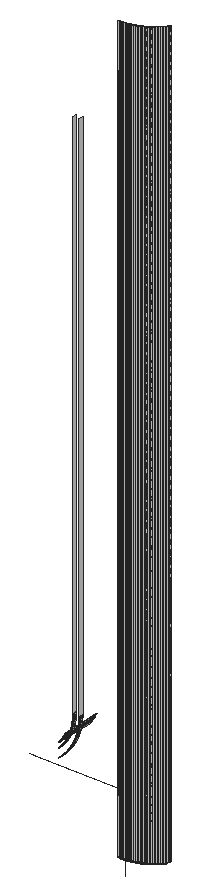
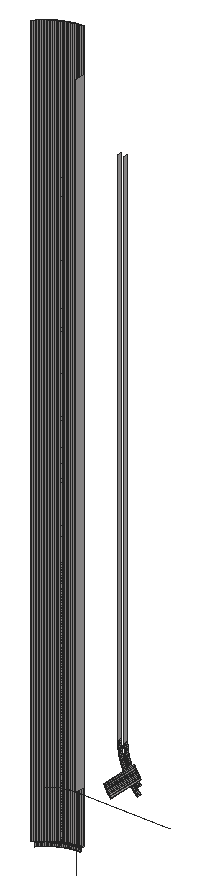
# SketchUp Ruby script. Lengths in inches.
U = 1.inch
M = Sketchup.active_model
def pt(a) = Geom::Point3d.new(a.map { |v| v * U })
def face(e, loops, mat)
  f = e.add_face(loops[0].map { |a| pt(a) })
  loops[1..].each { |l| e.add_face(l.map { |a| pt(a) }).erase! }
  f.material = f.back_material = mat if mat
  f
end
# faces: each face lists its corners as indices into pts; further lists are holes
def faces(e, pts, list, mat = nil) = list.each { |f| face(e, (f[0].is_a?(Array) ? f : [f]).map { |l| l.map { |i| pts[i] } }, mat) }
# xy, xz, yz: faces in a plane at the given z, y or x. An outline is a flat list of corners, or four numbers for a rectangle; further outlines are holes
def ring(l) = l.size == 4 ? [[l[0], l[1]], [l[2], l[1]], [l[2], l[3]], [l[0], l[3]]] : l.each_slice(2).to_a
def flat(e, list, mat, &to3) = list.each { |f| face(e, (f[0].is_a?(Array) ? f : [f]).map { |l| ring(l).map { |u, v| to3.(u, v) } }, mat) }
def xy(e, z, list, mat = nil) = flat(e, list, mat) { |x, y| [x, y, z] }
def xz(e, y, list, mat = nil) = flat(e, list, mat) { |x, z| [x, y, z] }
def yz(e, x, list, mat = nil) = flat(e, list, mat) { |y, z| [x, y, z] }
def lines(e, pts, list) = list.each { |a, b| e.add_line(pt(pts[a]), pt(pts[b])) }
# prism: a flat outline (further loops are holes) pulled along v
def prism(e, loops, v, mat = nil)
  f = face(e, loops, mat); d = Geom::Vector3d.new(v.map { |x| x * U })
  f.pushpull(f.normal.samedirection?(d) ? d.length : -d.length)
end
def box(e, o, s, mat = nil) = prism(e, [[o, [o[0] + s[0], o[1], o[2]], [o[0] + s[0], o[1] + s[1], o[2]], [o[0], o[1] + s[1], o[2]]]], [0, 0, s[2]], mat)
def at(x, y, z, deg = 0) = Geom::Transformation.translation(pt([x, y, z])) * Geom::Transformation.rotation(ORIGIN, Z_AXIS, deg.degrees)
def axes(o, x, y, z) = Geom::Transformation.new([*x, 0, *y, 0, *z, 0, *pt(o).to_a, 1])
def part(name) = M.definitions.add(name)
# library, detail: a bought-in or finely detailed component or shape, given as its bounding box
def library(name, o, s) = part(name).tap { |d| box(d.entities, o, s) }
def detail(e, o, s) = box(e.add_group.entities, o, s)
def put(e, d, t, mat = nil) = e.add_instance(d, t).tap { |i| i.material = mat if mat }
def group(e, t, mat = nil) = e.add_group.tap { |g| g.transformation = t; g.material = mat if mat }.entities
root = M.entities
M.materials.add("[Quartz Light Brown]").color = [215, 212, 212]
xz(root,143,[[480,133,480.2,368]],"[Quartz Light Brown]")
xz(root,143.01,[[480.39,133,480.59,368]],"[Quartz Light Brown]")
xz(root,144,[[480,132,480.18,133],[480.18,132,480.37,133]],"[Quartz Light Brown]")
yz(root,465.99,[[143,167.37,144.25,167.58]],"[Quartz Light Brown]")
yz(root,466,[[143,167.79,144.25,168],[143,168,144.25,336]],"[Quartz Light Brown]")
yz(root,467.99,[[143,167.29,144.25,167.53]],"[Quartz Light Brown]")
yz(root,468,[[143,167.76,144.25,168],[143,168,144.25,336]],"[Quartz Light Brown]")
yz(root,480,[[143,150,146,354]],"[Quartz Light Brown]")
p = [[480.37,144,133],[480.37,144,132],[480.55,144.01,132],[480.55,144.01,133],[480.73,144.02,132],[480.73,144.02,133],
  [480.92,144.03,132],[480.92,144.03,133],[481.1,144.04,132],[481.1,144.04,133],[481.28,144.06,132],[481.28,144.06,133],
  [481.46,144.08,132],[481.46,144.08,133],[481.65,144.1,132],[481.65,144.1,133],[481.83,144.12,132],[481.83,144.12,133],
  [482.01,144.14,132],[482.01,144.14,133],[482.19,144.17,132],[482.19,144.17,133],[482.37,144.2,132],[482.37,144.2,133],
  [482.55,144.23,132],[482.55,144.23,133],[482.73,144.27,132],[482.73,144.27,133],[482.91,144.31,132],[482.91,144.31,133],
  [483.09,144.35,132],[483.09,144.35,133],[483.27,144.39,132],[483.27,144.39,133],[483.45,144.43,132],[483.45,144.43,133],
  [483.625,144.48,132],[483.625,144.48,133],[483.8,144.53,132],[483.8,144.53,133],[483.98,144.58,132],[483.98,144.58,133],
  [484.15,144.63,132],[484.15,144.63,133],[484.33,144.69,132],[484.33,144.69,133],[484.5,144.74,132],[484.5,144.74,133],
  [484.67,144.8,132],[484.67,144.8,133],[484.85,144.87,132],[484.85,144.87,133],[485.02,144.93,132],[485.02,144.93,133],
  [485.1875,145,132],[485.1875,145,133],[485.36,145.07,132],[485.36,145.07,133],[485.53,145.14,132],[485.53,145.14,133],
  [485.69,145.21,132],[485.69,145.21,133],[485.86,145.29,132],[485.86,145.29,133],[486.03,145.36,132],[486.03,145.36,133],
  [486.19,145.44,132],[486.19,145.44,133],[486.36,145.53,132],[486.36,145.53,133],[486.52,145.61,132],[486.52,145.61,133],
  [486.68,145.7,132],[486.68,145.7,133],[486.84,145.79,132],[486.84,145.79,133],[487,145.875,132],[487,145.875,133],
  [487.16,145.97,132],[487.16,145.97,133],[487.31,146.0625,132],[487.31,146.0625,133],[487.47,146.16,132],[487.47,146.16,133],
  [487.625,146.26,132],[487.625,146.26,133],[487.78,146.36,132],[487.78,146.36,133],[487.93,146.46,132],[487.93,146.46,133],
  [488.08,146.57,132],[488.08,146.57,133],[488.23,146.67,132],[488.23,146.67,133],[488.375,146.78,132],[488.375,146.78,133],
  [488.52,146.89,132],[488.52,146.89,133],[488.67,147.01,132],[488.67,147.01,133],[488.81,147.12,132],[488.81,147.12,133],
  [488.95,147.24,132],[488.95,147.24,133],[489.09,147.35,132],[489.09,147.35,133],[489.23,147.47,132],[489.23,147.47,133],
  [489.37,147.6,132],[489.37,147.6,133],[489.5,147.72,132],[489.5,147.72,133],[489.64,147.84,132],[489.64,147.84,133],
  [489.77,147.97,132],[489.77,147.97,133],[489.9,148.1,132],[489.9,148.1,133],[490.03,148.23,132],[490.03,148.23,133],
  [490.16,148.36,132],[490.16,148.36,133],[490.28,148.5,132],[490.28,148.5,133],[490.4,148.63,132],[490.4,148.63,133],
  [490.53,148.77,132],[490.53,148.77,133],[490.65,148.91,132],[490.65,148.91,133],[490.76,149.05,132],[490.76,149.05,133],
  [480.2,143,368],[480.2,143,133],[480.39,143.01,133],[480.39,143.01,368],[480.59,143.01,368],[480.59,143.01,133],
  [480.79,143.02,133],[480.79,143.02,368],[480.98,143.03,133],[480.98,143.03,368],[481.18,143.05,133],[481.18,143.05,368],
  [481.37,143.0625,133],[481.37,143.0625,368],[481.57,143.08,133],[481.57,143.08,368],[481.76,143.1,133],[481.76,143.1,368],
  [481.96,143.13,133],[481.96,143.13,368],[482.15,143.16,133],[482.15,143.16,368],[482.35,143.18,133],[482.35,143.18,368],
  [482.54,143.22,133],[482.54,143.22,368],[482.73,143.25,133],[482.73,143.25,368],[482.93,143.29,133],[482.93,143.29,368],
  [483.12,143.33,133],[483.12,143.33,368],[483.31,143.37,133],[483.31,143.37,368],[483.5,143.41,133],[483.5,143.41,368],
  [483.69,143.46,133],[483.69,143.46,368],[483.88,143.51,133],[483.88,143.51,368],[484.07,143.5625,133],[484.07,143.5625,368],
  [484.26,143.62,133],[484.26,143.62,368],[484.45,143.67,133],[484.45,143.67,368],[484.64,143.73,133],[484.64,143.73,368],
  [484.82,143.8,133],[484.82,143.8,368],[485.01,143.86,133],[485.01,143.86,368],[485.19,143.93,133],[485.19,143.93,368],
  [485.375,144,133],[485.375,144,368],[485.56,144.07,133],[485.56,144.07,368],[485.74,144.14,133],[485.74,144.14,368],
  [485.92,144.22,133],[485.92,144.22,368],[486.1,144.3,133],[486.1,144.3,368],[486.28,144.38,133],[486.28,144.38,368],
  [486.46,144.46,133],[486.46,144.46,368],[486.63,144.55,133],[486.63,144.55,368],[486.81,144.63,133],[486.81,144.63,368],
  [486.98,144.73,133],[486.98,144.73,368],[487.16,144.82,133],[487.16,144.82,368],[487.33,144.91,133],[487.33,144.91,368],
  [487.5,145.01,133],[487.5,145.01,368],[487.67,145.11,133],[487.67,145.11,368],[487.84,145.21,133],[487.84,145.21,368],
  [488,145.3125,133],[488,145.3125,368],[488.17,145.42,133],[488.17,145.42,368],[488.33,145.53,133],[488.33,145.53,368],
  [488.5,145.64,133],[488.5,145.64,368],[488.66,145.75,133],[488.66,145.75,368],[488.82,145.86,133],[488.82,145.86,368],
  [488.97,145.98,133],[488.97,145.98,368],[489.13,146.1,133],[489.13,146.1,368],[489.29,146.22,133],[489.29,146.22,368],
  [489.44,146.34,133],[489.44,146.34,368],[489.59,146.47,133],[489.59,146.47,368],[489.74,146.59,133],[489.74,146.59,368],
  [489.89,146.72,133],[489.89,146.72,368],[490.04,146.85,133],[490.04,146.85,368],[490.18,146.99,133],[490.18,146.99,368],
  [490.33,147.12,133],[490.33,147.12,368],[490.47,147.26,133],[490.47,147.26,368],[490.61,147.39,133],[490.61,147.39,368],
  [490.74,147.53,133],[490.74,147.53,368],[490.88,147.67,133],[490.88,147.67,368],[491.01,147.82,133],[491.01,147.82,368],
  [491.15,147.96,133],[491.15,147.96,368],[491.28,148.11,133],[491.28,148.11,368],[491.41,148.26,133],[491.41,148.26,368],
  [491.53,148.41,133],[491.53,148.41,368],[491.66,148.56,133],[491.66,148.56,368],[491.78,148.71,133],[491.78,148.71,368],
  [491.9,148.87,133],[491.9,148.87,368],[492.02,149.03,133],[492.02,149.03,368],[461.69,144.25,154.3125],[461.69,143,154.3125],
  [461.87,143,154.47],[461.87,144.25,154.47],[462.04,143,154.625],[462.04,144.25,154.625],[462.22,143,154.78],[462.22,144.25,154.78],
  [462.39,143,154.94],[462.39,144.25,154.94],[462.56,143,155.11],[462.56,144.25,155.11],[462.73,143,155.27],[462.73,144.25,155.27],
  [462.89,143,155.44],[462.89,144.25,155.44],[463.06,143,155.61],[463.06,144.25,155.61],[463.22,143,155.78],[463.22,144.25,155.78],
  [463.375,143,155.96],[463.375,144.25,155.96],[463.53,143,156.13],[463.53,144.25,156.13],[463.6875,143,156.31],[463.6875,144.25,156.31],
  [463.84,143,156.49],[463.84,144.25,156.49],[463.99,143,156.67],[463.99,144.25,156.67],[464.14,143,156.86],[464.14,144.25,156.86],
  [464.28,143,157.04],[464.28,144.25,157.04],[461.75,143,157.14],[461.61,143,156.99],[461.61,144.25,156.99],[461.75,144.25,157.14],
  [464.42,143,157.23],[464.42,144.25,157.23],[461.89,143,157.29],[461.89,144.25,157.29],[464.5625,143,157.42],[464.5625,144.25,157.42],
  [462.03,143,157.45],[462.03,144.25,157.45],[464.7,143,157.61],[464.7,144.25,157.61],[462.17,143,157.61],[462.17,144.25,157.61],
  [462.3,143,157.77],[462.3,144.25,157.77],[464.83,143,157.8],[464.83,144.25,157.8],[462.43,143,157.93],[462.43,144.25,157.93],
  [464.97,143,158],[464.97,144.25,158],[462.57,143,158.09],[462.57,144.25,158.09],[465.1,143,158.2],[465.1,144.25,158.2],
  [462.69,143,158.26],[462.69,144.25,158.26],[465.22,143,158.39],[465.22,144.25,158.39],[462.82,143,158.43],[462.82,144.25,158.43],
  [462.94,143,158.6],[462.94,144.25,158.6],[465.35,143,158.6],[465.35,144.25,158.6],[461.66,143,158.56],[461.78,143,158.71],
  [461.78,155,158.71],[461.66,155,158.56],[463.07,143,158.77],[463.07,144.25,158.77],[465.47,143,158.8],[465.47,144.25,158.8],
  [461.9,143,158.87],[461.9,155,158.87],[463.1875,143,158.9375],[463.1875,144.25,158.9375],[465.59,143,159],[465.59,144.25,159],
  [462.02,143,159.03],[462.02,155,159.03],[463.3,143,159.11],[463.3,144.25,159.11],[462.14,143,159.18],[462.14,155,159.18],
  [465.7,143,159.2],[465.7,144.25,159.2],[463.42,143,159.29],[463.42,144.25,159.29],[462.25,143,159.34],[462.25,155,159.34],
  [465.82,143,159.41],[465.82,144.25,159.41],[462.36,143,159.5],[462.36,155,159.5],[463.53,143,159.46],[463.53,144.25,159.46],
  [465.93,143,159.62],[465.93,144.25,159.62],[462.47,143,159.67],[462.47,155,159.67],[463.64,143,159.64],[463.64,144.25,159.64],
  [463.75,143,159.82],[463.75,144.25,159.82],[466.04,143,159.83],[466.04,144.25,159.83],[462.58,143,159.83],[462.58,155,159.83],
  [462.6875,143,160],[462.6875,155,160],[463.86,143,160],[463.86,144.25,160],[466.14,143,160.04],[466.14,144.25,160.04],
  [462.79,143,160.16],[462.79,155,160.16],[463.96,143,160.18],[463.96,144.25,160.18],[466.25,143,160.25],[466.25,144.25,160.25],
  [462.89,143,160.33],[462.89,155,160.33],[464.0625,143,160.37],[464.0625,144.25,160.37],[462.99,143,160.5],[462.99,155,160.5],
  [466.35,143,160.46],[466.35,144.25,160.46],[464.16,143,160.55],[464.16,144.25,160.55],[463.09,143,160.67],[463.09,155,160.67],
  [466.44,143,160.68],[466.44,144.25,160.68],[464.26,143,160.74],[464.26,144.25,160.74],[463.18,143,160.84],[463.18,155,160.84],
  [464.35,143,160.92],[464.35,144.25,160.92],[466.54,143,160.89],[466.54,144.25,160.89],[463.27,143,161.02],[463.27,155,161.02],
  [464.44,143,161.11],[464.44,144.25,161.11],[466.63,143,161.11],[466.63,144.25,161.11],[463.37,143,161.19],[463.37,155,161.19],
  [464.53,143,161.3],[464.53,144.25,161.3],[466.72,143,161.33],[466.72,144.25,161.33],[463.45,143,161.37],[463.45,155,161.37],
  [464.62,143,161.49],[464.62,144.25,161.49],[466.8,143,161.55],[466.8,144.25,161.55],[463.54,143,161.54],[463.54,155,161.54],
  [463.62,143,161.72],[463.62,155,161.72],[464.7,143,161.68],[464.7,144.25,161.68],[466.89,143,161.77],[466.89,144.25,161.77],
  [463.7,143,161.9],[463.7,155,161.9],[464.78,143,161.88],[464.78,144.25,161.88],[466.97,143,161.99],[466.97,144.25,161.99],
  [463.78,143,162.08],[463.78,155,162.08],[464.86,143,162.07],[464.86,144.25,162.07],[467.04,143,162.21],[467.04,144.25,162.21],
  [464.9375,143,162.27],[464.9375,144.25,162.27],[467.12,143,162.4375],[467.12,144.25,162.4375],[465.01,143,162.46],[465.01,144.25,162.46],
  [467.19,143,162.66],[467.19,144.25,162.66],[465.08,143,162.66],[465.08,144.25,162.66],[465.15,143,162.86],[465.15,144.25,162.86],
  [467.26,143,162.89],[467.26,144.25,162.89],[465.22,143,163.06],[465.22,144.25,163.06],[467.32,143,163.11],[467.32,144.25,163.11],
  [465.28,143,163.26],[465.28,144.25,163.26],[467.39,143,163.34],[467.39,144.25,163.34],[465.34,143,163.46],[465.34,144.25,163.46],
  [467.45,143,163.57],[467.45,144.25,163.57],[465.4,143,163.66],[465.4,144.25,163.66],[467.5,143,163.8],[467.5,144.25,163.8],
  [465.45,143,163.86],[465.45,144.25,163.86],[467.56,143,164.03],[467.56,144.25,164.03],[465.51,143,164.0625],[465.51,144.25,164.0625],
  [467.61,143,164.26],[467.61,144.25,164.26],[465.56,143,164.26],[465.56,144.25,164.26],[465.61,143,164.47],[465.61,144.25,164.47],
  [467.65,143,164.49],[467.65,144.25,164.49],[465.65,143,164.67],[465.65,144.25,164.67],[467.7,143,164.72],[467.7,144.25,164.72],
  [465.69,143,164.88],[465.69,144.25,164.88],[467.74,143,164.95],[467.74,144.25,164.95],[465.73,143,165.08],[465.73,144.25,165.08],
  [467.78,143,165.18],[467.78,144.25,165.18],[465.77,143,165.29],[465.77,144.25,165.29],[467.8125,143,165.42],[467.8125,144.25,165.42],
  [465.8,143,165.5],[465.8,144.25,165.5],[467.85,143,165.65],[467.85,144.25,165.65],[465.83,143,165.7],[465.83,144.25,165.7],
  [465.86,143,165.91],[465.86,144.25,165.91],[467.875,143,165.88],[467.875,144.25,165.88],[465.89,143,166.12],[465.89,144.25,166.12],
  [467.9,143,166.12],[467.9,144.25,166.12],[465.91,143,166.33],[465.91,144.25,166.33],[467.92,143,166.35],[467.92,144.25,166.35],
  [465.93,143,166.54],[465.93,144.25,166.54],[467.94,143,166.59],[467.94,144.25,166.59],[465.95,143,166.74],[465.95,144.25,166.74],
  [467.96,143,166.82],[467.96,144.25,166.82],[465.97,143,166.95],[465.97,144.25,166.95],[467.98,143,167.06],[467.98,144.25,167.06],
  [465.98,143,167.16],[465.98,144.25,167.16],[467.99,143,167.29],[467.99,144.25,167.29],[465.99,143,167.37],[465.99,144.25,167.37],
  [467.99,144.25,167.53],[467.99,143,167.53],[468,143,167.76],[468,144.25,167.76],[466,143,167.79],[465.99,143,167.58],
  [465.99,144.25,167.58],[466,144.25,167.79],[480,146,150],[480,146,126],[450,146,150],[480.16,146,150],
  [480.3125,146,150],[480.47,146.01,150],[480.63,146.02,150],[480.78,146.03,150],[480.94,146.04,150],[481.1,146.05,150],
  [481.25,146.07,150],[481.41,146.08,150],[481.57,146.1,150],[481.72,146.125,150],[481.88,146.15,150],[482.03,146.17,150],
  [482.1875,146.2,150],[482.34,146.23,150],[482.49,146.26,150],[482.65,146.3,150],[482.8,146.33,150],[482.95,146.37,150],
  [483.11,146.41,150],[483.26,146.45,150],[483.41,146.49,150],[483.56,146.54,150],[483.71,146.59,150],[483.86,146.64,150],
  [484.01,146.6875,150],[484.15,146.74,150],[484.3,146.8,150],[484.45,146.85,150],[484.59,146.91,150],[484.74,146.97,150],
  [484.88,147.04,150],[485.02,147.1,150],[485.17,147.17,150],[485.31,147.24,150],[485.45,147.31,150],[485.59,147.38,150],
  [485.73,147.45,150],[485.86,147.53,150],[486,147.61,150],[486.14,147.6875,150],[486.27,147.77,150],[486.4,147.85,150],
  [486.54,147.9375,150],[486.67,148.02,150],[486.8,148.11,150],[486.93,148.2,150],[487.05,148.29,150],[487.18,148.38,150],
  [487.31,148.48,150],[487.43,148.58,150],[487.55,148.67,150],[487.67,148.77,150],[487.79,148.875,150],[487.91,148.98,150]]
faces(root,p,[[0,1,2,3],[3,2,4,5],[5,4,6,7],[7,6,8,9],[9,8,10,11],[11,10,12,13],[13,12,14,15],[15,14,16,17],
  [17,16,18,19],[19,18,20,21],[21,20,22,23],[23,22,24,25],[25,24,26,27],[27,26,28,29],[29,28,30,31],[31,30,32,33],
  [33,32,34,35],[35,34,36,37],[37,36,38,39],[39,38,40,41],[41,40,42,43],[43,42,44,45],[45,44,46,47],[47,46,48,49],
  [49,48,50,51],[51,50,52,53],[53,52,54,55],[55,54,56,57],[57,56,58,59],[59,58,60,61],[61,60,62,63],[63,62,64,65],
  [65,64,66,67],[67,66,68,69],[69,68,70,71],[71,70,72,73],[73,72,74,75],[75,74,76,77],[77,76,78,79],[79,78,80,81],
  [81,80,82,83],[83,82,84,85],[85,84,86,87],[87,86,88,89],[89,88,90,91],[91,90,92,93],[93,92,94,95],[95,94,96,97],
  [97,96,98,99],[99,98,100,101],[101,100,102,103],[103,102,104,105],[105,104,106,107],[107,106,108,109],[109,108,110,111],[111,110,112,113],
  [113,112,114,115],[115,114,116,117],[117,116,118,119],[119,118,120,121],[121,120,122,123],[123,122,124,125],[125,124,126,127],[127,126,128,129],
  [129,128,130,131],[132,133,134,135],[136,137,138,139],[139,138,140,141],[141,140,142,143],[143,142,144,145],[145,144,146,147],[147,146,148,149],
  [149,148,150,151],[151,150,152,153],[153,152,154,155],[155,154,156,157],[157,156,158,159],[159,158,160,161],[161,160,162,163],[163,162,164,165],
  [165,164,166,167],[167,166,168,169],[169,168,170,171],[171,170,172,173],[173,172,174,175],[175,174,176,177],[177,176,178,179],[179,178,180,181],
  [181,180,182,183],[183,182,184,185],[185,184,186,187],[187,186,188,189],[189,188,190,191],[191,190,192,193],[193,192,194,195],[195,194,196,197],
  [197,196,198,199],[199,198,200,201],[201,200,202,203],[203,202,204,205],[205,204,206,207],[207,206,208,209],[209,208,210,211],[211,210,212,213],
  [213,212,214,215],[215,214,216,217],[217,216,218,219],[219,218,220,221],[221,220,222,223],[223,222,224,225],[225,224,226,227],[227,226,228,229],
  [229,228,230,231],[231,230,232,233],[233,232,234,235],[235,234,236,237],[237,236,238,239],[239,238,240,241],[241,240,242,243],[243,242,244,245],
  [245,244,246,247],[247,246,248,249],[249,248,250,251],[251,250,252,253],[253,252,254,255],[255,254,256,257],[257,256,258,259],[259,258,260,261],
  [261,260,262,263],[263,262,264,265],[265,264,266,267],[267,266,268,269],[269,268,270,271],[271,270,272,273],[274,275,276,277],[277,276,278,279],
  [279,278,280,281],[281,280,282,283],[283,282,284,285],[285,284,286,287],[287,286,288,289],[289,288,290,291],[291,290,292,293],[293,292,294,295],
  [295,294,296,297],[297,296,298,299],[299,298,300,301],[301,300,302,303],[303,302,304,305],[305,304,306,307],[308,309,310,311],[307,306,312,313],
  [314,308,311,315],[313,312,316,317],[318,314,315,319],[317,316,320,321],[322,318,319,323],[324,322,323,325],[321,320,326,327],[328,324,325,329],
  [327,326,330,331],[332,328,329,333],[331,330,334,335],[336,332,333,337],[335,334,338,339],[340,336,337,341],[342,340,341,343],[339,338,344,345],
  [346,347,348,349],[350,342,343,351],[345,344,352,353],[347,354,355,348],[356,350,351,357],[353,352,358,359],[354,360,361,355],[362,356,357,363],
  [360,364,365,361],[359,358,366,367],[368,362,363,369],[364,370,371,365],[367,366,372,373],[370,374,375,371],[376,368,369,377],[373,372,378,379],
  [374,380,381,375],[382,376,377,383],[384,382,383,385],[379,378,386,387],[380,388,389,381],[388,390,391,389],[392,384,385,393],[387,386,394,395],
  [390,396,397,391],[398,392,393,399],[395,394,400,401],[396,402,403,397],[404,398,399,405],[402,406,407,403],[401,400,408,409],[410,404,405,411],
  [406,412,413,407],[409,408,414,415],[416,410,411,417],[412,418,419,413],[420,416,417,421],[415,414,422,423],[418,424,425,419],[426,420,421,427],
  [423,422,428,429],[424,430,431,425],[432,426,427,433],[429,428,434,435],[430,436,437,431],[438,432,433,439],[435,434,440,441],[436,442,443,437],
  [442,444,445,443],[446,438,439,447],[441,440,448,449],[444,450,451,445],[452,446,447,453],[449,448,454,455],[450,456,457,451],[458,452,453,459],
  [455,454,460,461],[462,458,459,463],[461,460,464,465],[466,462,463,467],[465,464,468,469],[470,466,467,471],[472,470,471,473],[469,468,474,475],
  [476,472,473,477],[475,474,478,479],[480,476,477,481],[479,478,482,483],[484,480,481,485],[483,482,486,487],[488,484,485,489],[487,486,490,491],
  [492,488,489,493],[491,490,494,495],[496,492,493,497],[495,494,498,499],[500,496,497,501],[502,500,501,503],[499,498,504,505],[506,502,503,507],
  [505,504,508,509],[510,506,507,511],[509,508,512,513],[514,510,511,515],[513,512,516,517],[518,514,515,519],[517,516,520,521],[522,518,519,523],
  [521,520,524,525],[526,522,523,527],[528,526,527,529],[525,524,530,531],[532,528,529,533],[531,530,534,535],[536,532,533,537],[535,534,538,539],
  [540,536,537,541],[539,538,542,543],[544,540,541,545],[543,542,546,547],[548,544,545,549],[547,546,550,551],[552,548,549,553],[551,550,554,555],
  [556,552,553,557],[558,559,560,561],[562,563,564,565]],"[Quartz Light Brown]")
lines(root,p,[[566,567],[568,566],[566,569],[569,570],[570,571],[571,572],[572,573],[573,574],[574,575],[575,576],[576,577],[577,578],
  [578,579],[579,580],[580,581],[581,582],[582,583],[583,584],[584,585],[585,586],[586,587],[587,588],[588,589],[589,590],
  [590,591],[591,592],[592,593],[593,594],[594,595],[595,596],[596,597],[597,598],[598,599],[599,600],[600,601],[601,602],
  [602,603],[603,604],[604,605],[605,606],[606,607],[607,608],[608,609],[609,610],[610,611],[611,612],[612,613],[613,614],
  [614,615],[615,616],[616,617],[617,618],[618,619],[619,620],[620,621],[621,622],[622,623]])
